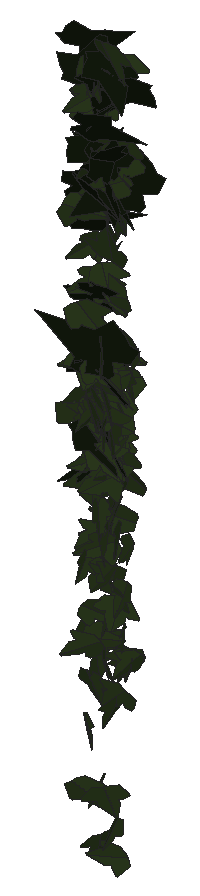
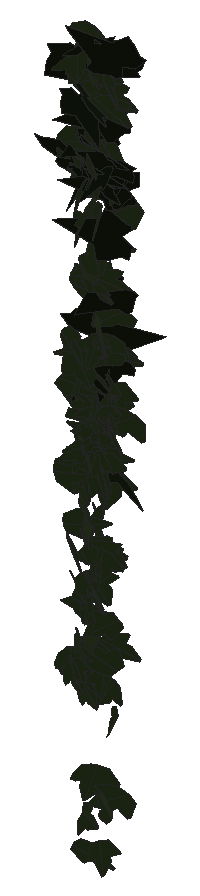
# SketchUp Ruby script. Lengths in inches.
U = 1.inch
M = Sketchup.active_model
def pt(a) = Geom::Point3d.new(a.map { |v| v * U })
def face(e, loops, mat)
  f = e.add_face(loops[0].map { |a| pt(a) })
  loops[1..].each { |l| e.add_face(l.map { |a| pt(a) }).erase! }
  f.material = f.back_material = mat if mat
  f
end
# faces: each face lists its corners as indices into pts; further lists are holes
def faces(e, pts, list, mat = nil) = list.each { |f| face(e, (f[0].is_a?(Array) ? f : [f]).map { |l| l.map { |i| pts[i] } }, mat) }
# xy, xz, yz: faces in a plane at the given z, y or x. An outline is a flat list of corners, or four numbers for a rectangle; further outlines are holes
def ring(l) = l.size == 4 ? [[l[0], l[1]], [l[2], l[1]], [l[2], l[3]], [l[0], l[3]]] : l.each_slice(2).to_a
def flat(e, list, mat, &to3) = list.each { |f| face(e, (f[0].is_a?(Array) ? f : [f]).map { |l| ring(l).map { |u, v| to3.(u, v) } }, mat) }
def xy(e, z, list, mat = nil) = flat(e, list, mat) { |x, y| [x, y, z] }
def xz(e, y, list, mat = nil) = flat(e, list, mat) { |x, z| [x, y, z] }
def yz(e, x, list, mat = nil) = flat(e, list, mat) { |y, z| [x, y, z] }
def lines(e, pts, list) = list.each { |a, b| e.add_line(pt(pts[a]), pt(pts[b])) }
# prism: a flat outline (further loops are holes) pulled along v
def prism(e, loops, v, mat = nil)
  f = face(e, loops, mat); d = Geom::Vector3d.new(v.map { |x| x * U })
  f.pushpull(f.normal.samedirection?(d) ? d.length : -d.length)
end
def box(e, o, s, mat = nil) = prism(e, [[o, [o[0] + s[0], o[1], o[2]], [o[0] + s[0], o[1] + s[1], o[2]], [o[0], o[1] + s[1], o[2]]]], [0, 0, s[2]], mat)
def at(x, y, z, deg = 0) = Geom::Transformation.translation(pt([x, y, z])) * Geom::Transformation.rotation(ORIGIN, Z_AXIS, deg.degrees)
def axes(o, x, y, z) = Geom::Transformation.new([*x, 0, *y, 0, *z, 0, *pt(o).to_a, 1])
def part(name) = M.definitions.add(name)
# library, detail: a bought-in or finely detailed component or shape, given as its bounding box
def library(name, o, s) = part(name).tap { |d| box(d.entities, o, s) }
def detail(e, o, s) = box(e.add_group.entities, o, s)
def put(e, d, t, mat = nil) = e.add_instance(d, t).tap { |i| i.material = mat if mat }
def group(e, t, mat = nil) = e.add_group.tap { |g| g.transformation = t; g.material = mat if mat }.entities
root = M.entities
M.materials.add("1026 AP 7946 SUNNY SIDE UP").color = [254, 231, 186]
M.materials.add("efeu1").color = [18, 25, 13]
M.materials.add("efeu2").color = [43, 57, 29]
c1 = part("ivyleaf_9")
p = [[1.54,2.16,1.25],[1.36,2.04,1.19],[-0.21,0.99,0.68],[-0.71,1.11,0.82],[-0.85,0.86,0.67],[-0.8,0.17,0.21],
  [-0.9,-0.01,0.1],[-0.67,-0.16,-0.02],[-0.08,-0.08,-0.05],[-0.03,-0.6,-0.4],[0.65,-0.88,-0.66],[0.83,-0.6,-0.49],
  [1.29,-0.42,-0.43],[1.8125,-0.07,-0.26],[1.21,0.44,0.15]]
faces(c1.entities,p,[[0,1,2,3,4,5,6,7,8,9,10,11,12,13,14]],"efeu1")
c2 = part("ivyleaf_10")
p = [[0,0.5,-0.03],[-0.0625,2.02,-0.43],[-0.19,2.01,-0.46],[-0.54,1.05,-0.29],[-0.52,0.625,-0.18],[-0.83,0.76,-0.28],
  [-1.16,0.64,-0.33],[-1.15,0.33,-0.24],[-0.77,-0.39,0.02],[-0.3,-0.51,0.16],[0.04,-0.48,0.23],[-0.02,2.01,-0.4375],
  [-0.06,2.01,-0.43],[0.04,-0.49,0.23],[0.67,-0.49,0.14],[1.38,0.36,-0.2],[1.375,0.51,-0.24],[0.81,0.65,-0.19],
  [0.62,0.59,-0.15],[0.6,1.09,-0.28],[0.5,1.23,-0.31]]
faces(c2.entities,p,[[0,1,2,3,4,5,6,7,8,9,10],[11,12,0,13,14,15,16,17,18,19,20]],"efeu2")
put(root,c1,axes([145.29,212.73,260.21],[-0.23592,0.19622,-0.03429],[0.01278,-0.03699,-0.25415],[-0.31297,-0.14942,0.01546]),"1026 AP 7946 SUNNY SIDE UP")
put(root,c2,axes([145.27,213.03,258.8125],[-0.19175,-0.0597,0.17107],[-0.15112,-0.14727,-0.12786],[0.2333,-0.14446,0.05778]),"1026 AP 7946 SUNNY SIDE UP")
put(root,c2,axes([144.95,212.7,261.08],[-0.30513,-0.04958,-0.16532],[0.26366,-0.06018,-0.19042],[-0.00303,-0.24433,0.07887]),"1026 AP 7946 SUNNY SIDE UP")
put(root,c2,axes([145.28,212.72,256.99],[-0.11524,-0.07436,0.18577],[-0.16296,-0.14888,-0.10726],[0.26056,-0.126,0.01508]),"1026 AP 7946 SUNNY SIDE UP")
put(root,c2,axes([145.16,212.71,261.49],[-0.11336,-0.23366,-0.0521],[0.04249,0.04313,-0.25131],[0.37306,-0.07591,0.01279]),"1026 AP 7946 SUNNY SIDE UP")
put(root,c2,axes([144.97,212.59,264.75],[-0.09028,-0.09873,-0.22337],[0.26916,0.13721,-0.11055],[0.2594,-0.17674,0.03697]),"1026 AP 7946 SUNNY SIDE UP")
put(root,c2,axes([145.28,212.83,266.75],[0.17794,0.10489,-0.19645],[-0.2344,-0.12016,-0.15943],[-0.25046,0.18698,0.00964]),"1026 AP 7946 SUNNY SIDE UP")
put(root,c2,axes([145.06,212.9375,260.94],[0.2182,-0.15308,0.12202],[0.12583,-0.0885,-0.21337],[0.27804,0.16019,0.0008]),"1026 AP 7946 SUNNY SIDE UP")
put(root,c2,axes([145.27,212.96,260.35],[0.17427,-0.13251,-0.17175],[-0.12993,0.14555,-0.17571],[0.30763,0.13654,0.02309]),"1026 AP 7946 SUNNY SIDE UP")
put(root,c2,axes([145.26,212.83,264.11],[0.05826,0.09489,-0.2181],[-0.19146,-0.17518,-0.1036],[-0.31143,0.12544,0.02289]),"1026 AP 7946 SUNNY SIDE UP")
put(root,c2,axes([145.21,213.02,258.7],[-0.32789,-0.00546,0.01212],[-0.01749,-0.0232,-0.21374],[0.01058,-0.20757,0.02234]),"1026 AP 7946 SUNNY SIDE UP")
put(root,c2,axes([145.29,212.86,267.13],[0.19947,-0.15217,-0.15619],[-0.14632,0.11866,-0.20337],[0.30337,0.15728,0.00461]),"1026 AP 7946 SUNNY SIDE UP")
put(root,c2,axes([144.99,213.08,256.87],[-0.18272,-0.05275,0.17179],[0.23147,0.07928,0.13174],[-0.14934,0.18742,-0.006]),"1026 AP 7946 SUNNY SIDE UP")
put(root,c2,axes([145.2,212.92,260.32],[-0.09349,-0.22092,-0.0492],[0.02098,0.04456,-0.23542],[0.35436,-0.06092,0.00096]),"1026 AP 7946 SUNNY SIDE UP")
put(root,c2,axes([145.27,212.91,266.66],[0.32023,0.03996,-0.13682],[-0.19442,-0.05544,-0.21248],[-0.09954,0.23686,-0.02515]),"1026 AP 7946 SUNNY SIDE UP")
put(root,c1,axes([144.91,212.92,267.46],[-0.01134,-0.03135,0.26133],[0.39958,-0.02976,0.00348],[0.04574,0.25221,0.03441]),"1026 AP 7946 SUNNY SIDE UP")
put(root,c2,axes([145.34,212.91,262.67],[-0.05927,0.11504,0.19613],[-0.24856,0.12112,-0.1073],[-0.24481,-0.15082,0.06146]),"1026 AP 7946 SUNNY SIDE UP")
put(root,c2,axes([145.22,213.01,258.75],[-0.11801,0.17078,0.08731],[-0.08076,0.06853,-0.19091],[-0.288,-0.0892,0.01776]),"1026 AP 7946 SUNNY SIDE UP")
put(root,c1,axes([144.9375,212.9,264.4],[0.14939,0.17131,-0.17672],[0.11349,0.15699,0.20247],[0.36504,-0.11892,0.00937]),"1026 AP 7946 SUNNY SIDE UP")
put(root,c2,axes([145.19,212.7,258.48],[0.02582,0.13628,-0.1563],[-0.0454,-0.14991,-0.14209],[-0.31836,0.03243,0.00759]),"1026 AP 7946 SUNNY SIDE UP")
put(root,c2,axes([145.22,212.94,256.59],[0.03205,0.20038,0.04882],[-0.08094,0.04997,-0.19937],[-0.31307,0.00759,0.05654]),"1026 AP 7946 SUNNY SIDE UP")
put(root,c2,axes([145.24,213.07,260.14],[-0.02459,-0.21021,0.09933],[0.0315,-0.0987,-0.21623],[0.36307,-0.00567,0.02549]),"1026 AP 7946 SUNNY SIDE UP")
put(root,c2,axes([145.34,212.75,261.17],[-0.19657,-0.16843,0.11652],[-0.08362,-0.10216,-0.21605],[0.30872,-0.13491,0.01567]),"1026 AP 7946 SUNNY SIDE UP")
put(root,c2,axes([145.42,212.7,262.06],[-0.0488,-0.02049,0.23248],[-0.21878,-0.17821,-0.03741],[0.28146,-0.14207,0.01123]),"1026 AP 7946 SUNNY SIDE UP")
put(root,c2,axes([145.05,212.73,254.37],[-0.22182,-0.02669,-0.1729],[0.26619,-0.00534,-0.14588],[0.02053,-0.21907,0.02332]),"1026 AP 7946 SUNNY SIDE UP")
put(root,c2,axes([145.11,212.87,257.48],[0.12032,0.06741,0.18092],[0.0966,0.16983,-0.09394],[-0.27898,0.08788,0.0455]),"1026 AP 7946 SUNNY SIDE UP")
put(root,c2,axes([145.19,212.87,254.12],[0.11805,-0.18919,0.05072],[-0.01623,0.04998,0.20979],[-0.30739,-0.0753,0.0084]),"1026 AP 7946 SUNNY SIDE UP")
put(root,c2,axes([145.25,213.02,264.77],[-0.17207,0.20116,0.03516],[-0.04946,0.02033,-0.23509],[-0.31669,-0.11247,0.01761]),"1026 AP 7946 SUNNY SIDE UP")
put(root,c2,axes([145.1875,212.84,267.27],[0.12729,0.23152,-0.05299],[-0.02189,-0.05101,-0.25295],[-0.37273,0.08206,-0.00324]),"1026 AP 7946 SUNNY SIDE UP")
put(root,c2,axes([145.19,212.81,256.33],[-0.28535,0.07925,-0.06327],[0.07471,-0.04489,-0.2031],[-0.13931,-0.1864,0.02067]),"1026 AP 7946 SUNNY SIDE UP")
put(root,c2,axes([145.38,212.84,263.48],[0.18951,0.05158,-0.19038],[-0.24474,-0.10191,-0.13426],[-0.17716,0.19596,-0.01817]),"1026 AP 7946 SUNNY SIDE UP")
put(root,c2,axes([145.24,212.75,259.91],[-0.22715,-0.19167,-0.01082],[0.07686,-0.02536,-0.241],[0.29179,-0.14253,0.05506]),"1026 AP 7946 SUNNY SIDE UP")
put(root,c1,axes([145.14,212.97,265.58],[0.28779,-0.1235,-0.10871],[-0.14721,0.04842,-0.22689],[0.20786,0.20528,-0.01018]),"1026 AP 7946 SUNNY SIDE UP")
put(root,c1,axes([145.08,212.98,265.72],[-0.13555,-0.12335,-0.19574],[0.2146,0.13305,-0.15256],[0.28314,-0.15989,0.02192]),"1026 AP 7946 SUNNY SIDE UP")
put(root,c2,axes([145.29,212.91,253.46],[-0.09402,-0.19271,-0.0229],[0.00736,0.02067,-0.20774],[0.30474,-0.05996,-0.00205]),"1026 AP 7946 SUNNY SIDE UP")
put(root,c2,axes([145.4,212.78,260.29],[0.09275,0.02895,-0.20925],[-0.2269,-0.14462,-0.0652],[-0.22969,0.15456,-0.02009]),"1026 AP 7946 SUNNY SIDE UP")
put(root,c2,axes([145.23,213.11,263.86],[-0.00966,-0.23363,-0.07576],[-0.00554,-0.07214,0.24034],[-0.38447,0.00691,-0.00156]),"1026 AP 7946 SUNNY SIDE UP")
put(root,c2,axes([145.3,213.07,258.17],[-0.06984,0.12268,0.16115],[0.02798,-0.15648,0.13131],[0.31047,0.0417,0.02442]),"1026 AP 7946 SUNNY SIDE UP")
put(root,c2,axes([145.47,212.63,261.3],[-0.02623,-0.00116,-0.23208],[-0.21071,0.18162,0.01033],[0.28473,0.1343,-0.01374]),"1026 AP 7946 SUNNY SIDE UP")
put(root,c2,axes([145.29,212.82,261.15],[0.00684,-0.11654,0.20774],[0.03544,-0.20119,-0.12107],[0.36541,0.02169,0.00786]),"1026 AP 7946 SUNNY SIDE UP")
put(root,c2,axes([145.44,212.93,258.73],[0.11992,0.05819,-0.20752],[-0.25338,-0.12143,-0.09954],[-0.21172,0.17828,0.00158]),"1026 AP 7946 SUNNY SIDE UP")
put(root,c1,axes([145.28,212.67,267.11],[-0.30976,-0.02031,0.1742],[0.26218,0.03054,0.20394],[-0.05544,0.25789,-0.00889]),"1026 AP 7946 SUNNY SIDE UP")
put(root,c2,axes([145.41,213,258.23],[-0.19788,-0.15269,0.10939],[-0.08074,-0.09579,-0.20349],[0.28189,-0.13462,0.01851]),"1026 AP 7946 SUNNY SIDE UP")
put(root,c2,axes([145.26,212.98,261.22],[0.25321,0.14081,-0.03166],[-0.02074,-0.03269,-0.21997],[-0.22595,0.1608,-0.01529]),"1026 AP 7946 SUNNY SIDE UP")
put(root,c1,axes([145.01,212.66,265.09],[0.19151,0.04626,0.23141],[0.35316,0.02594,-0.13096],[-0.07095,0.25397,-0.02723]),"1026 AP 7946 SUNNY SIDE UP")
put(root,c1,axes([145.71,212.6,262.26],[-0.07354,0.04445,0.34091],[-0.48694,0.11847,-0.06083],[-0.19523,-0.31224,0.02332]),"1026 AP 7946 SUNNY SIDE UP")
put(root,c2,axes([145.25,212.63,255.65],[-0.09487,0.17424,-0.08891],[0.0419,-0.08314,-0.19043],[-0.30356,-0.06593,0.0015]),"1026 AP 7946 SUNNY SIDE UP")
put(root,c2,axes([145.17,213.125,257.95],[0.1704,-0.15077,-0.10663],[0.1151,-0.07341,0.19026],[-0.26268,-0.12997,0.0142]),"1026 AP 7946 SUNNY SIDE UP")
put(root,c1,axes([145.14,212.65,263.3],[0.34993,0.08467,0.04804],[0.07929,-0.00325,-0.2444],[-0.12924,0.22725,-0.01988]),"1026 AP 7946 SUNNY SIDE UP")
put(root,c1,axes([145.06,212.67,265.15],[0.33406,-0.11031,0.07127],[0.07929,-0.05364,-0.24574],[0.18934,0.2171,-0.02283]),"1026 AP 7946 SUNNY SIDE UP")
put(root,c2,axes([145.32,212.63,261.33],[-0.22479,0.1867,-0.01001],[-0.00747,-0.01718,-0.2419],[-0.29396,-0.14233,0.0138]),"1026 AP 7946 SUNNY SIDE UP")
put(root,c2,axes([145.24,212.73,261.28],[0.11911,0.13997,0.18041],[0.04141,0.17719,-0.15732],[-0.34909,0.06878,0.04289]),"1026 AP 7946 SUNNY SIDE UP")
put(root,c2,axes([145.33,212.95,262.41],[-0.06959,-0.17026,-0.13464],[0.05831,0.12437,-0.18046],[0.33149,-0.05762,0.00348]),"1026 AP 7946 SUNNY SIDE UP")
put(root,c2,axes([145.43,212.82,261.66],[-0.35983,0.03232,0.05435],[-0.08827,-0.02513,-0.23595],[-0.04031,-0.23345,0.03151]),"1026 AP 7946 SUNNY SIDE UP")
put(root,c2,axes([145.11,212.69,262.89],[0.26561,0.07063,0.16494],[0.23619,0.05457,-0.18821],[-0.14006,0.22597,-0.00458]),"1026 AP 7946 SUNNY SIDE UP")
put(root,c1,axes([145.35,212.64,262.0625],[0.1948,0.21514,-0.03408],[-0.01553,-0.03388,-0.25581],[-0.34221,0.124,-0.00779]),"1026 AP 7946 SUNNY SIDE UP")
put(root,c2,axes([145.27,212.83,262.05],[0.283,0.11936,-0.07317],[0.07585,0.05648,0.22191],[0.20538,-0.18532,0.01887]),"1026 AP 7946 SUNNY SIDE UP")
put(root,c2,axes([145.29,213.21,257.33],[0.03978,-0.09099,0.18591],[0.10989,-0.16726,-0.09768],[0.29895,0.07359,0.01117]),"1026 AP 7946 SUNNY SIDE UP")
put(root,c2,axes([145.3,212.63,262.13],[0.33303,0.11502,-0.0185],[-0.01395,-0.02258,-0.2479],[-0.18267,0.21141,-0.0148]),"1026 AP 7946 SUNNY SIDE UP")
put(root,c2,axes([145.11,212.98,256.93],[0.10511,-0.03425,-0.19469],[0.28867,-0.04671,0.07542],[-0.08771,-0.19475,0.01491]),"1026 AP 7946 SUNNY SIDE UP")
put(root,c2,axes([145.375,212.66,265.69],[-0.07307,-0.20485,-0.14525],[0.04936,0.13626,-0.2156],[0.38686,-0.05608,0.00007]),"1026 AP 7946 SUNNY SIDE UP")
put(root,c2,axes([145.3125,212.82,260.4],[0.19597,0.18873,0.02836],[0.00663,0.02888,-0.23249],[-0.29959,0.12409,0.01341]),"1026 AP 7946 SUNNY SIDE UP")
put(root,c2,axes([145.4,212.78,260.4],[-0.0239,0.06781,-0.20864],[-0.07231,-0.1997,-0.06637],[-0.32854,0.03902,0.02979]),"1026 AP 7946 SUNNY SIDE UP")
put(root,c2,axes([145.33,213.16,259.08],[-0.01903,-0.03747,-0.22392],[0.02238,-0.21715,0.03652],[-0.34576,-0.012,0.01469]),"1026 AP 7946 SUNNY SIDE UP")
put(root,c2,axes([145.3,212.72,262.32],[-0.24857,-0.12201,-0.11176],[0.17176,0.03193,-0.20207],[0.18983,-0.18866,0.03648]),"1026 AP 7946 SUNNY SIDE UP")
put(root,c1,axes([145.68,212.8,265.63],[-0.09929,0.10633,0.22178],[-0.26013,0.14122,-0.12136],[-0.27246,-0.17358,0.03505]),"1026 AP 7946 SUNNY SIDE UP")
put(root,c2,axes([145.34,213,261.14],[0.03023,-0.10713,0.1977],[0.12229,-0.1775,-0.1108],[0.32411,0.07696,0.02337]),"1026 AP 7946 SUNNY SIDE UP")
put(root,c2,axes([145.36,212.8,259.42],[-0.00659,0.23155,-0.06431],[-0.01361,-0.06385,-0.23875],[-0.37738,-0.00174,0.00974]),"1026 AP 7946 SUNNY SIDE UP")
put(root,c2,axes([145.32,213.125,263.7],[0.00701,-0.17242,-0.15715],[0.04163,-0.1502,0.17594],[-0.35856,-0.02081,0.01735]),"1026 AP 7946 SUNNY SIDE UP")
put(root,c1,axes([145.25,212.67,260.84],[0.10427,-0.22079,-0.0987],[-0.00245,0.0977,-0.23556],[0.37766,0.06159,0.02572]),"1026 AP 7946 SUNNY SIDE UP")
put(root,c2,axes([145.53,212.71,260.89],[-0.1164,0.19284,0.1053],[-0.18288,0.05527,-0.19598],[-0.28945,-0.11247,0.08148]),"1026 AP 7946 SUNNY SIDE UP")
put(root,c2,axes([145.44,212.88,267.29],[0.04349,-0.23379,0.09035],[0.02905,-0.08742,-0.24291],[0.39228,0.03239,0.00797]),"1026 AP 7946 SUNNY SIDE UP")
put(root,c1,axes([145.47,213.06,266.75],[-0.28657,0.02648,-0.16473],[0.20696,-0.11659,-0.17495],[-0.14912,-0.21269,0.07375]),"1026 AP 7946 SUNNY SIDE UP")
put(root,c2,axes([145.55,212.93,260.29],[-0.19163,0.17924,0.05827],[-0.17013,-0.01301,-0.2014],[-0.24107,-0.1333,0.09581]),"1026 AP 7946 SUNNY SIDE UP")
put(root,c2,axes([145.66,213.11,259.16],[-0.04633,-0.03045,-0.21374],[-0.31092,-0.06518,0.03844],[-0.10895,0.19898,-0.0188]),"1026 AP 7946 SUNNY SIDE UP")
put(root,c2,axes([145.23,212.8,267.12],[0.10168,-0.036,0.25314],[0.29662,-0.15835,-0.07591],[0.25448,0.19896,-0.01267]),"1026 AP 7946 SUNNY SIDE UP")
put(root,c2,axes([145.43,212.98,261.39],[-0.24726,0.17314,-0.02204],[0.00527,-0.02711,-0.24057],[-0.27445,-0.1565,0.01524]),"1026 AP 7946 SUNNY SIDE UP")
put(root,c2,axes([145.53,213.16,262.12],[-0.22107,-0.15502,0.06666],[-0.05208,-0.0583,-0.21546],[0.2595,-0.14377,0.01354]),"1026 AP 7946 SUNNY SIDE UP")
put(root,c2,axes([145.5625,212.8125,267.07],[-0.36393,-0.0756,0.07342],[-0.09325,-0.04804,-0.24966],[0.13471,-0.23749,0.02554]),"1026 AP 7946 SUNNY SIDE UP")
put(root,c2,axes([145.41,212.96,265.69],[0.02321,-0.17065,0.1678],[0.08757,-0.15705,-0.17459],[0.36153,0.049,0.03152]),"1026 AP 7946 SUNNY SIDE UP")
put(root,c1,axes([145.61,213.02,266.67],[-0.05137,0.23838,-0.04436],[-0.00386,-0.04513,-0.24799],[-0.38126,-0.03166,0.00849]),"1026 AP 7946 SUNNY SIDE UP")
put(root,c2,axes([145.51,213.02,264.59],[-0.08784,0.19685,0.11204],[-0.06663,0.09967,-0.20986],[-0.34643,-0.06908,0.01195]),"1026 AP 7946 SUNNY SIDE UP")
put(root,c2,axes([145.54,213,257.86],[-0.26365,0.13532,0.02568],[-0.06827,-0.01598,-0.21831],[-0.20508,-0.16865,0.03966]),"1026 AP 7946 SUNNY SIDE UP")
put(root,c2,axes([145.54,213,261.1],[0.30737,0.01904,-0.08116],[-0.11963,-0.02863,-0.20149],[-0.04441,0.20885,-0.01897]),"1026 AP 7946 SUNNY SIDE UP")
put(root,c2,axes([145.66,212.78,265.31],[0.2868,-0.02555,-0.17511],[-0.26708,0.00982,-0.18939],[0.03996,0.24903,-0.00903]),"1026 AP 7946 SUNNY SIDE UP")
put(root,c2,axes([145.7,212.85,253.28],[0.13138,-0.04188,-0.18664],[-0.28321,0.03008,-0.09268],[0.07117,0.19701,-0.02429]),"1026 AP 7946 SUNNY SIDE UP")
put(root,c2,axes([145.63,212.66,260.08],[0.284,-0.02962,-0.13735],[-0.21174,-0.00342,-0.18741],[0.03426,0.22437,-0.01965]),"1026 AP 7946 SUNNY SIDE UP")
put(root,c2,axes([145.55,213.02,260.33],[-0.34348,-0.0521,0.01011],[-0.0077,-0.02288,-0.23046],[0.08309,-0.21747,0.02046]),"1026 AP 7946 SUNNY SIDE UP")
put(root,c1,axes([145.67,212.8,265.1875],[-0.38473,-0.03,0.01189],[-0.01363,-0.0251,-0.25291],[0.04877,-0.24367,0.02313]),"1026 AP 7946 SUNNY SIDE UP")
put(root,c2,axes([145.43,212.83,263.64],[0.15414,0.20508,0.01257],[0.0204,0.00602,-0.23395],[-0.32229,0.09846,-0.0088]),"1026 AP 7946 SUNNY SIDE UP")
put(root,c1,axes([145.22,212.61,266.26],[0.28602,0.04058,0.17131],[0.26383,0.00399,-0.19033],[-0.0514,0.24627,-0.02366]),"1026 AP 7946 SUNNY SIDE UP")
put(root,c2,axes([145.48,213.08,260.51],[0.13632,0.17597,-0.06939],[-0.02891,-0.06699,-0.20208],[-0.29543,0.08776,-0.01224]),"1026 AP 7946 SUNNY SIDE UP")
put(root,c2,axes([145.8,212.77,263.33],[-0.12382,0.04338,0.22808],[-0.35433,-0.01196,-0.08032],[-0.00484,-0.23444,0.04488]),"1026 AP 7946 SUNNY SIDE UP")
put(root,c1,axes([145.43,212.92,265.26],[-0.23196,-0.06741,-0.18486],[0.27753,0.03933,-0.16482],[0.11612,-0.22865,0.02466]),"1026 AP 7946 SUNNY SIDE UP")
put(root,c2,axes([145.75,212.88,261.21],[0.11779,0.07359,0.21284],[-0.2639,-0.12061,0.10646],[0.22103,-0.18323,0.01369]),"1026 AP 7946 SUNNY SIDE UP")
put(root,c2,axes([145.63,213.05,257.13],[-0.12217,0.19095,0.02714],[-0.1431,-0.01239,-0.19198],[-0.26693,-0.08075,0.0905]),"1026 AP 7946 SUNNY SIDE UP")
put(root,c2,axes([145.73,213.16,261.69],[0.13861,0.01438,-0.19339],[-0.28383,-0.0528,-0.09176],[-0.08462,0.20064,-0.00903]),"1026 AP 7946 SUNNY SIDE UP")
put(root,c2,axes([145.5,212.76,261.49],[-0.15202,0.18571,-0.08001],[0.04226,-0.07466,-0.21589],[-0.31434,-0.09985,0.00967]),"1026 AP 7946 SUNNY SIDE UP")
put(root,c2,axes([145.6,212.78,260.125],[0.31599,0.03293,0.06981],[-0.11051,0.01384,0.20844],[0.04194,-0.21157,0.02323]),"1026 AP 7946 SUNNY SIDE UP")
put(root,c2,axes([145.54,213.03,259.46],[0.16428,-0.17437,0.06946],[0.04478,-0.06263,-0.20964],[0.2911,0.10804,-0.00695]),"1026 AP 7946 SUNNY SIDE UP")
put(root,c2,axes([145.64,212.62,256.82],[-0.16871,0.14107,0.10701],[-0.11486,0.07365,-0.18176],[-0.24955,-0.12927,0.01132]),"1026 AP 7946 SUNNY SIDE UP")
put(root,c2,axes([145.39,212.95,260.79],[0.28113,0.07014,0.10712],[0.16375,0.01664,-0.1967],[-0.10896,0.20596,-0.01923]),"1026 AP 7946 SUNNY SIDE UP")
put(root,c2,axes([145.74,212.44,258.89],[0.05094,-0.01212,0.24373],[-0.27359,0.16093,0.03397],[-0.25294,-0.17651,0.01234]),"1026 AP 7946 SUNNY SIDE UP")
put(root,c2,axes([145.62,212.95,265.95],[-0.38538,-0.00698,0.00545],[-0.00722,-0.02502,-0.25143],[0.01177,-0.24387,0.0242]),"1026 AP 7946 SUNNY SIDE UP")
put(root,c2,axes([145.52,213.08,260.62],[0.07109,0.19918,0.00402],[0.00822,0.00166,-0.21034],[-0.31311,0.04527,-0.00461]),"1026 AP 7946 SUNNY SIDE UP")
put(root,c2,axes([145.62,213.18,256.65],[-0.06645,-0.19412,0.04882],[0.007,-0.05046,-0.20441],[0.31454,-0.03989,0.01486]),"1026 AP 7946 SUNNY SIDE UP")
put(root,c2,axes([145.42,212.76,262.27],[0.05531,-0.03323,0.25208],[0.25246,-0.18497,-0.0507],[0.29541,0.1643,-0.00387]),"1026 AP 7946 SUNNY SIDE UP")
put(root,c2,axes([145.7,212.77,260.5],[0.12906,0.01195,0.21639],[-0.20017,0.18225,0.04164],[-0.26325,-0.13272,0.07443]),"1026 AP 7946 SUNNY SIDE UP")
put(root,c2,axes([145.47,212.59,262.07],[0.21682,0.1361,0.14808],[0.10489,0.13201,-0.19497],[-0.29212,0.14842,0.03991]),"1026 AP 7946 SUNNY SIDE UP")
put(root,c2,axes([145.62,212.89,260.11],[-0.00627,0.02988,0.22038],[0.03712,-0.21244,0.0298],[0.33733,0.02393,0.00081]),"1026 AP 7946 SUNNY SIDE UP")
put(root,c2,axes([145.58,212.98,257.68],[0.33685,0.00727,-0.00271],[-0.00267,-0.02802,-0.2191],[-0.01188,0.2124,-0.02754]),"1026 AP 7946 SUNNY SIDE UP")
put(root,c2,axes([145.57,212.75,267.67],[-0.3369,0.10995,-0.09017],[0.1093,-0.0571,-0.24774],[-0.19277,-0.22454,0.01713]),"1026 AP 7946 SUNNY SIDE UP")
put(root,c1,axes([145.62,212.55,265.57],[-0.0726,-0.06867,0.25643],[0.23969,0.19734,0.08624],[-0.32845,0.15919,0.00625]),"1026 AP 7946 SUNNY SIDE UP")
put(root,c2,axes([145.42,212.86,261.58],[0.27995,-0.0578,-0.15419],[0.23237,-0.02674,0.192],[-0.09701,-0.23084,0.01492]),"1026 AP 7946 SUNNY SIDE UP")
put(root,c2,axes([145.59,213.16,261.76],[-0.19132,0.14179,-0.09967],[0.06434,-0.09221,-0.19119],[-0.26286,-0.12577,0.02575]),"1026 AP 7946 SUNNY SIDE UP")
put(root,c2,axes([145.42,212.86,263.37],[0.22337,0.01494,0.18161],[0.27799,-0.0168,-0.14547],[0.00591,0.22571,-0.02152]),"1026 AP 7946 SUNNY SIDE UP")
put(root,c2,axes([145.69,212.89,259.87],[-0.03123,-0.20881,0.01746],[0.00055,-0.01825,-0.21618],[0.32957,-0.01975,0.00201]),"1026 AP 7946 SUNNY SIDE UP")
put(root,c1,axes([145.78,212.71,267.2],[0.24546,0.17173,-0.22477],[-0.2003,-0.17936,-0.23932],[-0.38929,0.20057,-0.01859]),"1026 AP 7946 SUNNY SIDE UP")
put(root,c2,axes([145.69,212.82,253.86],[-0.03126,0.1626,-0.13136],[-0.09107,-0.12824,-0.15877],[-0.31282,0.02109,0.05935]),"1026 AP 7946 SUNNY SIDE UP")
put(root,c2,axes([145.71,212.63,264.11],[-0.37976,0.04633,-0.00331],[-0.00113,0.01469,0.25301],[0.07305,0.2411,-0.01331]),"1026 AP 7946 SUNNY SIDE UP")
put(root,c2,axes([145.52,212.92,265.28],[-0.24172,0.04474,-0.17647],[0.18913,-0.14049,-0.1496],[-0.2048,-0.18255,0.07013]),"1026 AP 7946 SUNNY SIDE UP")
put(root,c1,axes([145.56,212.49,265.8125],[0.19672,0.15552,0.17332],[0.17117,0.12717,-0.20484],[-0.31583,0.16579,-0.00306]),"1026 AP 7946 SUNNY SIDE UP")
put(root,c2,axes([145.8,212.96,265.68],[0.3156,-0.02087,-0.14212],[-0.21755,-0.00013,-0.20752],[0.02693,0.24348,-0.01086]),"1026 AP 7946 SUNNY SIDE UP")
put(root,c2,axes([145.47,212.9,262.23],[-0.07406,-0.08584,-0.20348],[0.30431,0.07078,-0.07901],[0.14696,-0.18982,0.06106]),"1026 AP 7946 SUNNY SIDE UP")
put(root,c1,axes([145.76,212.83,260.3125],[0.07427,-0.20364,0.12691],[-0.01466,0.12509,0.21542],[-0.3749,-0.04524,0.01672]),"1026 AP 7946 SUNNY SIDE UP")
put(root,c2,axes([145.66,212.6,254.53],[-0.24725,-0.15557,-0.05592],[0.091,0.01682,-0.22595],[0.24208,-0.16521,0.02782]),"1026 AP 7946 SUNNY SIDE UP")
put(root,c2,axes([145.64,213.16,256.7],[0.21102,-0.15437,0.02633],[0.0592,-0.00199,-0.20891],[0.23904,0.13676,0.02849]),"1026 AP 7946 SUNNY SIDE UP")
put(root,c2,axes([145.72,213.09,256.8],[-0.1888,-0.16123,0.0283],[0.01315,-0.0412,-0.20486],[0.25708,-0.1163,0.03126]),"1026 AP 7946 SUNNY SIDE UP")
put(root,c2,axes([145.71,212.72,260.83],[-0.07824,0.21674,0.06081],[-0.0859,0.04571,-0.22477],[-0.34209,-0.06105,0.04253]),"1026 AP 7946 SUNNY SIDE UP")
put(root,c2,axes([145.55,212.6,260.55],[0.17539,0.17596,0.1075],[0.10635,0.07925,-0.21373],[-0.30274,0.12978,-0.0128]),"1026 AP 7946 SUNNY SIDE UP")
put(root,c2,axes([145.75,213.0625,258.75],[0.16526,-0.17073,-0.05904],[-0.05376,0.04509,-0.20621],[0.27754,0.1104,-0.00478]),"1026 AP 7946 SUNNY SIDE UP")
put(root,c2,axes([145.61,212.95,259.04],[0.1054,-0.13578,0.15352],[0.14507,-0.11987,-0.15518],[0.28286,0.11207,0.02238]),"1026 AP 7946 SUNNY SIDE UP")
put(root,c1,axes([145.66,212.58,261.87],[0.34396,-0.01389,-0.14481],[-0.21455,0.04567,-0.22326],[0.05695,0.25593,0.03353]),"1026 AP 7946 SUNNY SIDE UP")
put(root,c2,axes([145.66,213.03,267.35],[0.15979,0.21988,-0.04545],[-0.0225,-0.04335,-0.24974],[-0.3523,0.10249,-0.00466]),"1026 AP 7946 SUNNY SIDE UP")
put(root,c2,axes([145.87,212.99,262.33],[0.11902,-0.04935,-0.21362],[-0.18784,0.17207,-0.08622],[0.27706,0.13786,0.03332]),"1026 AP 7946 SUNNY SIDE UP")
put(root,c1,axes([145.65,212.6875,265.28],[0.27256,-0.14108,-0.16534],[-0.20914,0.08919,-0.22939],[0.26176,0.21816,-0.01111]),"1026 AP 7946 SUNNY SIDE UP")
put(root,c2,axes([145.7,212.82,265.04],[-0.11943,0.23108,0.01176],[-0.01533,0.00743,-0.25044],[-0.36337,-0.07626,0.0067]),"1026 AP 7946 SUNNY SIDE UP")
put(root,c2,axes([145.76,212.72,256.1],[-0.0003,-0.20331,0.07475],[0.00223,-0.07371,-0.20987],[0.34004,0.0003,0.00144]),"1026 AP 7946 SUNNY SIDE UP")
put(root,c1,axes([145.62,212.73,267.47],[-0.04882,-0.24541,-0.07578],[0.01858,0.07125,-0.25441],[0.4018,-0.03311,0.00256]),"1026 AP 7946 SUNNY SIDE UP")
put(root,c2,axes([145.96,213.02,259.9375],[-0.10675,0.06794,-0.19639],[-0.26069,0.09735,0.09694],[0.18351,0.17782,0.02347]),"1026 AP 7946 SUNNY SIDE UP")
put(root,c2,axes([145.81,213.11,256.74],[-0.07195,-0.12982,0.15605],[-0.02827,-0.15284,-0.14075],[0.31329,-0.04361,0.02314]),"1026 AP 7946 SUNNY SIDE UP")
put(root,c1,axes([146.16,212.8,265.32],[-0.19098,0.14071,0.29487],[-0.36852,0.16711,-0.18664],[-0.33849,-0.26133,0.03682]),"1026 AP 7946 SUNNY SIDE UP")
put(root,c2,axes([145.92,212.66,256.35],[-0.25231,-0.00564,0.12812],[-0.19091,-0.03798,-0.16334],[0.04349,-0.19945,0.02627]),"1026 AP 7946 SUNNY SIDE UP")
put(root,c2,axes([145.71,212.95,258.02],[0.26364,-0.13354,0.05823],[0.04898,-0.0524,-0.22008],[0.22317,0.16926,-0.02049]),"1026 AP 7946 SUNNY SIDE UP")
